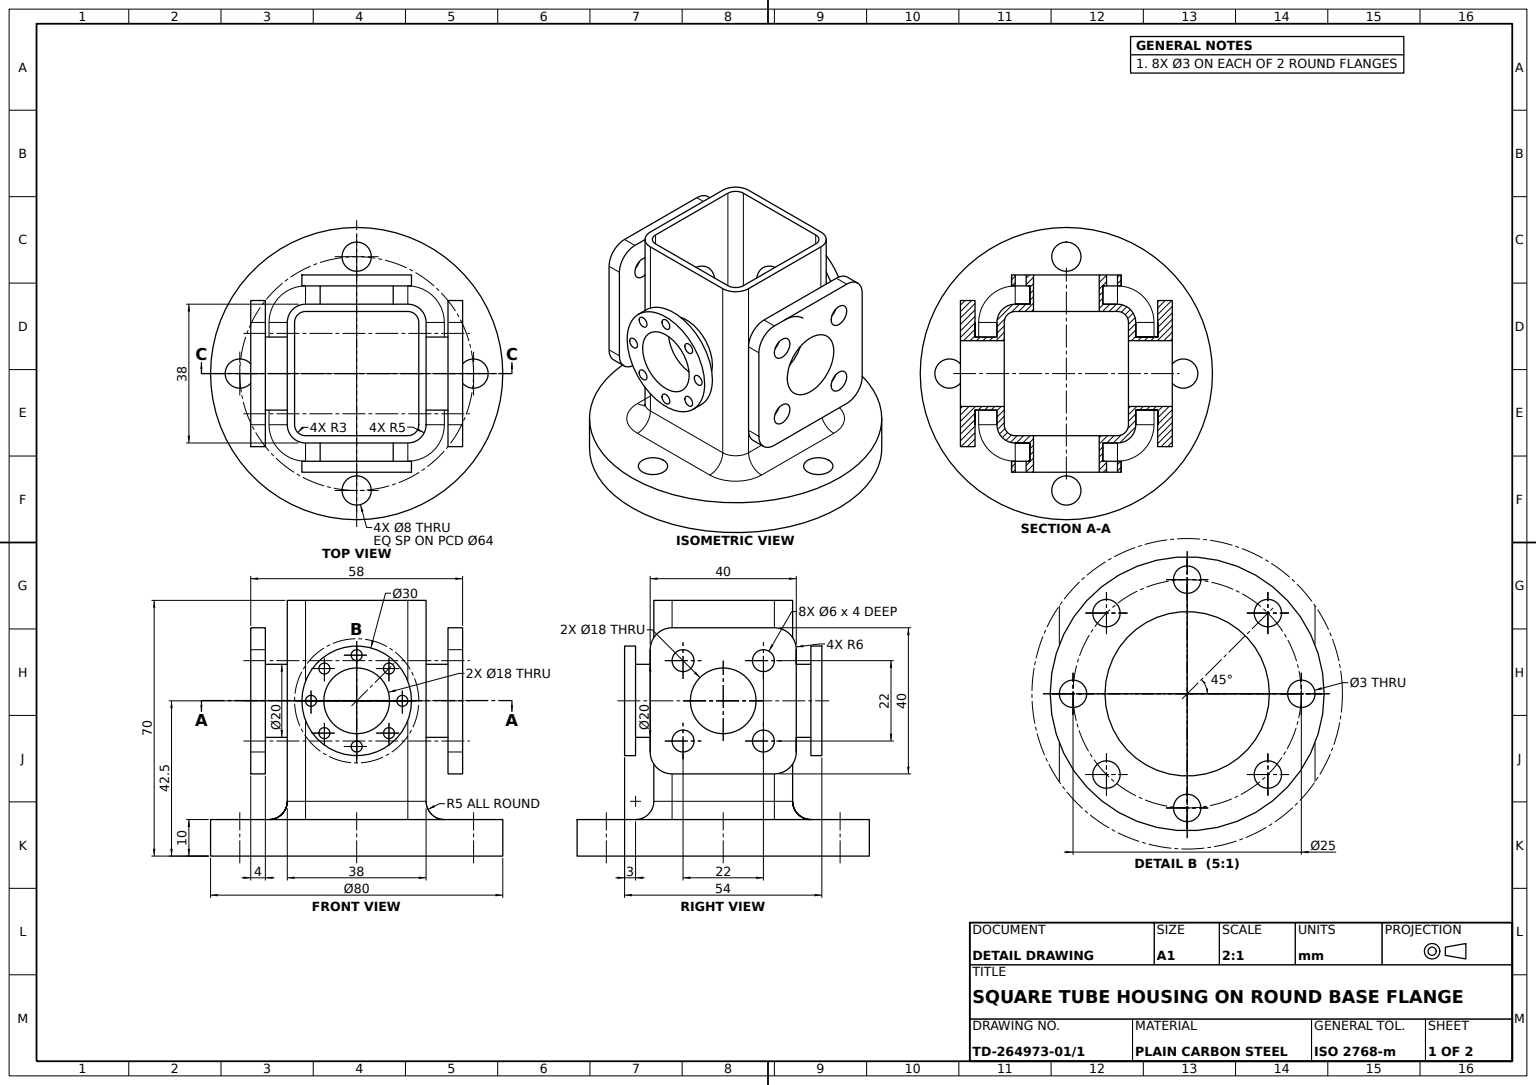
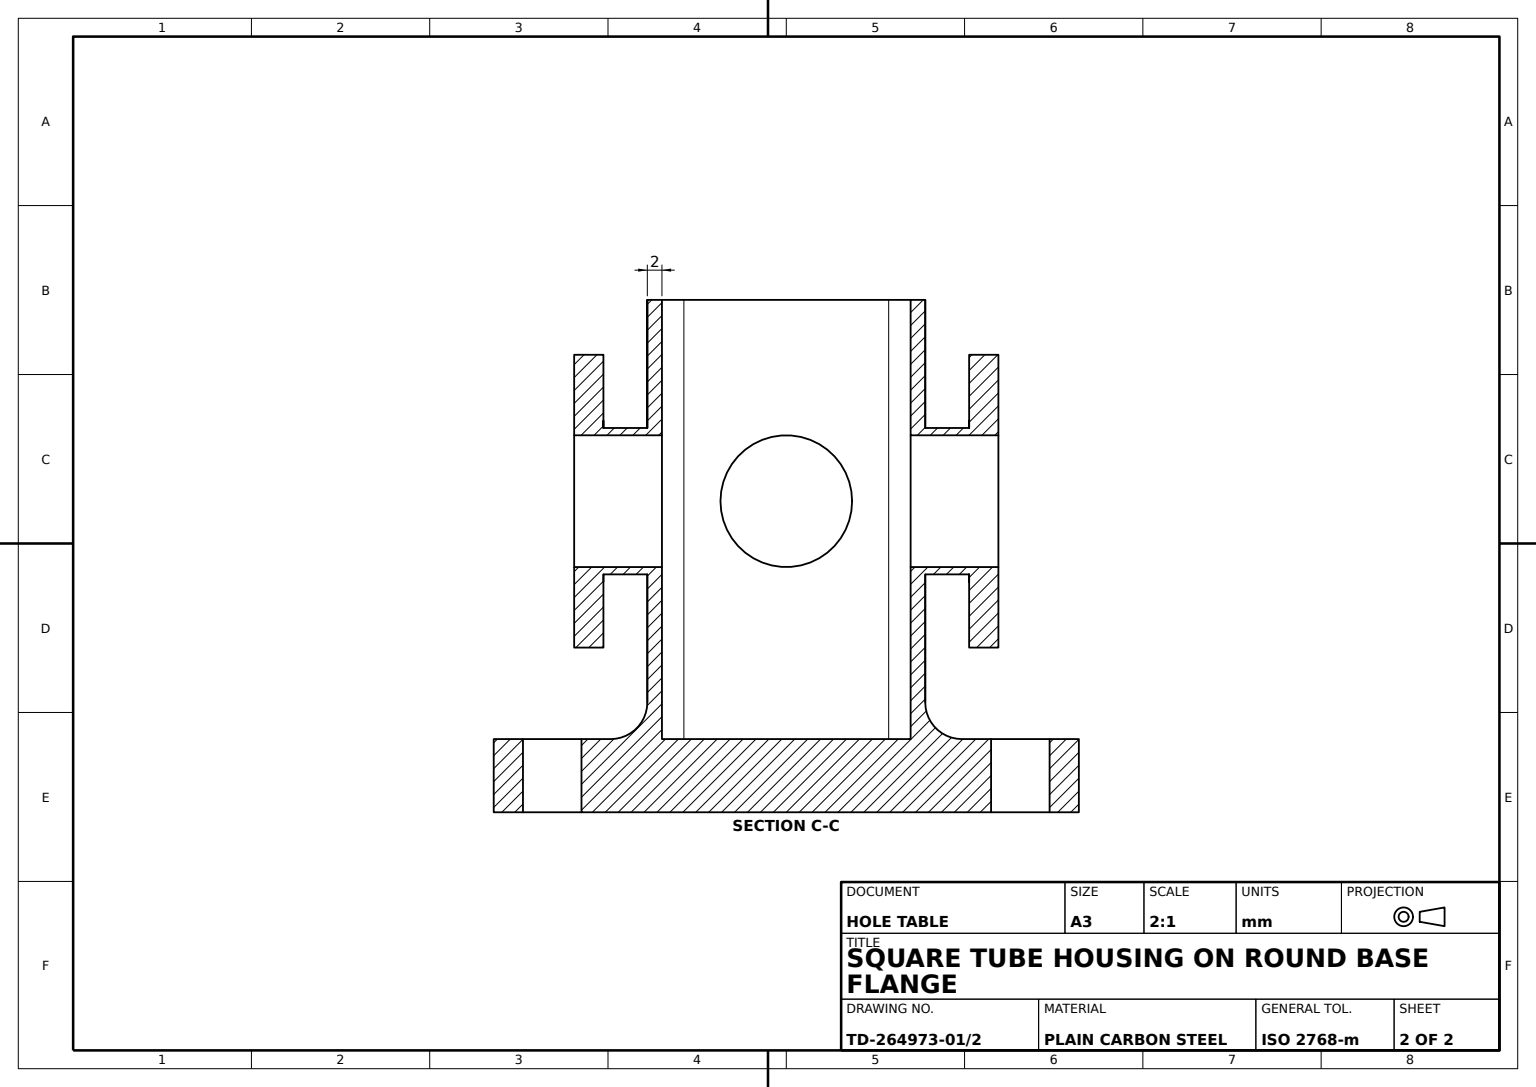
solid
v1 (29,42.5,-9)
v2 (29,42.5,9)
e1 v1 v2 CIRCLE(AX(P(29,42.5,0),D(1,0,0),D(0,0,-1)),9)
v3 (17,42.5,9)
e2 v2 v3 LINE
v4 (17,42.5,-9)
e3 v3 v4 CIRCLE(AX(P(17,42.5,0),D(-1,0,0),D(0,0,1)),9)
e4 v1 v4 LINE
face CYL(AX(P(41,42.5,0),D(-1,0,0),D(0,0,1)),9) rev [e1 e2 e3 -e4]
v5 (1.5,55,-27)
v6 (1.5,55,-24)
e5 v5 v6 LINE
v7 (-1.5,55,-24)
e6 v7 v6 CIRCLE(AX(P(0,55,-24),D(0,0,-1),D(-1,0,0)),1.5)
v8 (-1.5,55,-27)
e7 v8 v7 LINE
e8 v8 v5 CIRCLE(AX(P(0,55,-27),D(0,0,-1),D(-1,0,0)),1.5)
face CYL(AX(P(0,55,-27),D(0,0,1),D(1,0,0)),1.5) rev [e5 -e6 -e7 e8]
v9 (7.338835,51.338835,27)
v10 (7.338835,51.338835,24)
e9 v9 v10 LINE
v11 (10.338835,51.338835,24)
e10 v11 v10 CIRCLE(AX(P(8.838835,51.338835,24),D(0,0,1),D(1,0,0)),1.5)
v12 (10.338835,51.338835,27)
e11 v12 v11 LINE
e12 v12 v9 CIRCLE(AX(P(8.838835,51.338835,27),D(0,0,1),D(1,0,0)),1.5)
face CYL(AX(P(8.838835,51.338835,27),D(0,0,-1),D(-1,0,0)),1.5) rev [e9 -e10 -e11 e12]
v13 (-17,70,-14)
v14 (-17,70,14)
e13 v13 v14 LINE
v15 (-17,10,14)
e14 v14 v15 LINE
v16 (-17,10,-14)
e15 v16 v15 LINE
e16 v13 v16 LINE
v17 (-17,42.5,-9)
v18 (-17,42.5,9)
e17 v17 v18 CIRCLE(AX(P(-17,42.5,0),D(1,0,0),D(0,0,-1)),9)
e18 v18 v17 CIRCLE(AX(P(-17,42.5,0),D(1,0,0),D(0,0,-1)),9)
face PLANE(AX(P(-17,70,-14),D(1,0,0),D(0,0,-1))) [e13 e14 -e15 -e16] [-e17 -e18]
v19 (-25,62.5,-14)
v20 (-25,56.5,-20)
e19 v19 v20 CIRCLE(AX(P(-25,56.5,-14),D(-1,0,0),D(0,0,1)),6)
v21 (-29,56.5,-20)
e20 v21 v20 LINE
v22 (-29,62.5,-14)
e21 v22 v21 CIRCLE(AX(P(-29,56.5,-14),D(-1,0,0),D(0,0,1)),6)
e22 v22 v19 LINE
face CYL(AX(P(-29,56.5,-14),D(1,0,0),D(0,0,-1)),6) [e19 -e20 -e21 e22]
v23 (-1.5,30,-24)
v24 (1.5,30,-24)
e23 v23 v24 CIRCLE(AX(P(0,30,-24),D(0,0,-1),D(-1,0,0)),1.5)
v25 (-1.5,30,-27)
e24 v25 v23 LINE
v26 (1.5,30,-27)
e25 v25 v26 CIRCLE(AX(P(0,30,-27),D(0,0,-1),D(-1,0,0)),1.5)
e26 v26 v24 LINE
face CYL(AX(P(0,30,-27),D(0,0,1),D(1,0,0)),1.5) rev [-e23 -e24 e25 e26]
v27 (-25,42.5,-10)
v28 (-19,42.5,-10)
e27 v27 v28 LINE
v29 (-25,42.5,10)
e28 v29 v27 CIRCLE(AX(P(-25,42.5,0),D(-1,0,0),D(0,0,1)),10)
v30 (-19,42.5,10)
e29 v29 v30 LINE
e30 v30 v28 CIRCLE(AX(P(-19,42.5,0),D(-1,0,0),D(0,0,-1)),10)
face CYL(AX(P(-25,42.5,0),D(1,0,0),D(0,0,-1)),10) [-e27 -e28 e29 e30]
v31 (0,10,40)
v32 (0,0,40)
e31 v31 v32 LINE
v33 (0,0,-40)
e32 v32 v33 CIRCLE(AX(P(0,0,0),D(0,1,0),D(0,0,1)),40)
v34 (0,10,-40)
e33 v34 v33 LINE
e34 v31 v34 CIRCLE(AX(P(0,10,0),D(0,1,0),D(0,0,1)),40)
face CYL(AX(P(0,10,0),D(0,-1,0),D(0,0,-1)),40) [e31 e32 -e33 -e34]
v35 (0,10,28)
v36 (0,10,36)
e35 v35 v36 CIRCLE(AX(P(0,10,32),D(0,1,0),D(0,0,1)),4)
v37 (0,0,36)
e36 v36 v37 LINE
v38 (0,0,28)
e37 v38 v37 CIRCLE(AX(P(0,0,32),D(0,1,0),D(0,0,1)),4)
e38 v35 v38 LINE
face CYL(AX(P(0,10,32),D(0,-1,0),D(0,0,-1)),4) rev [e35 e36 -e37 -e38]
v39 (1.5,30,27)
v40 (1.5,30,24)
e39 v39 v40 LINE
v41 (-1.5,30,27)
e40 v39 v41 CIRCLE(AX(P(0,30,27),D(0,0,1),D(1,0,0)),1.5)
v42 (-1.5,30,24)
e41 v41 v42 LINE
e42 v40 v42 CIRCLE(AX(P(0,30,24),D(0,0,1),D(1,0,0)),1.5)
face CYL(AX(P(0,30,27),D(0,0,-1),D(-1,0,0)),1.5) rev [-e39 e40 e41 -e42]
v43 (-14,10,-17)
e43 v43 v16 CIRCLE(AX(P(-14,10,-14),D(0,1,0),D(1,0,0)),3)
v44 (-14,70,-17)
e44 v44 v43 LINE
e45 v44 v13 CIRCLE(AX(P(-14,70,-14),D(0,1,0),D(1,0,0)),3)
face CYL(AX(P(-14,70,-14),D(0,-1,0),D(0,0,-1)),3) rev [-e43 -e44 e45 e16]
v45 (29,62.5,14)
v46 (29,56.5,20)
e46 v45 v46 CIRCLE(AX(P(29,56.5,14),D(1,0,0),D(0,0,-1)),6)
v47 (25,62.5,14)
e47 v45 v47 LINE
v48 (25,56.5,20)
e48 v47 v48 CIRCLE(AX(P(25,56.5,14),D(1,0,0),D(0,0,-1)),6)
e49 v46 v48 LINE
face CYL(AX(P(29,56.5,14),D(-1,0,0),D(0,0,1)),6) [-e46 e47 e48 -e49]
v49 (-14,42.5,27)
v50 (-11,42.5,27)
e50 v49 v50 CIRCLE(AX(P(-12.5,42.5,27),D(0,0,1),D(1,0,0)),1.5)
v51 (-11,42.5,24)
e51 v50 v51 LINE
v52 (-14,42.5,24)
e52 v52 v51 CIRCLE(AX(P(-12.5,42.5,24),D(0,0,1),D(1,0,0)),1.5)
e53 v49 v52 LINE
face CYL(AX(P(-12.5,42.5,27),D(0,0,-1),D(-1,0,0)),1.5) rev [e50 e51 -e52 -e53]
v53 (-7.338835,51.338835,27)
v54 (-10.338835,51.338835,27)
e54 v53 v54 CIRCLE(AX(P(-8.838835,51.338835,27),D(0,0,1),D(1,0,0)),1.5)
v55 (-10.338835,51.338835,24)
e55 v54 v55 LINE
v56 (-7.338835,51.338835,24)
e56 v56 v55 CIRCLE(AX(P(-8.838835,51.338835,24),D(0,0,1),D(1,0,0)),1.5)
e57 v53 v56 LINE
face CYL(AX(P(-8.838835,51.338835,27),D(0,0,-1),D(-1,0,0)),1.5) rev [e54 e55 -e56 -e57]
v57 (11,42.5,-27)
v58 (11,42.5,-24)
e58 v57 v58 LINE
v59 (14,42.5,-24)
e59 v59 v58 CIRCLE(AX(P(12.5,42.5,-24),D(0,0,-1),D(-1,0,0)),1.5)
v60 (14,42.5,-27)
e60 v60 v59 LINE
e61 v60 v57 CIRCLE(AX(P(12.5,42.5,-27),D(0,0,-1),D(-1,0,0)),1.5)
face CYL(AX(P(12.5,42.5,-27),D(0,0,1),D(1,0,0)),1.5) rev [e58 -e59 -e60 e61]
v61 (-25,28.5,-20)
v62 (-25,22.5,-14)
e62 v61 v62 CIRCLE(AX(P(-25,28.5,-14),D(-1,0,0),D(0,0,1)),6)
v63 (-29,22.5,-14)
e63 v63 v62 LINE
v64 (-29,28.5,-20)
e64 v64 v63 CIRCLE(AX(P(-29,28.5,-14),D(-1,0,0),D(0,0,1)),6)
e65 v64 v61 LINE
face CYL(AX(P(-29,28.5,-14),D(1,0,0),D(0,0,-1)),6) [e62 -e63 -e64 e65]
v65 (29,53.5,14)
v66 (29,53.5,8)
e66 v65 v66 CIRCLE(AX(P(29,53.5,11),D(1,0,0),D(0,0,-1)),3)
v67 (25,53.5,8)
e67 v66 v67 LINE
v68 (25,53.5,14)
e68 v68 v67 CIRCLE(AX(P(25,53.5,11),D(1,0,0),D(0,0,-1)),3)
e69 v65 v68 LINE
face CYL(AX(P(29,53.5,11),D(-1,0,0),D(0,0,1)),3) rev [e66 e67 -e68 -e69]
v69 (25,28.5,20)
e70 v48 v69 LINE
v70 (29,28.5,20)
e71 v70 v69 LINE
e72 v46 v70 LINE
face PLANE(AX(P(29,56.5,20),D(0,0,-1),D(-1,0,0))) rev [e49 e70 -e71 -e72]
v71 (-25,28.5,20)
v72 (-25,56.5,20)
e73 v71 v72 LINE
v73 (-29,56.5,20)
e74 v73 v72 LINE
v74 (-29,28.5,20)
e75 v74 v73 LINE
e76 v74 v71 LINE
face PLANE(AX(P(-29,56.5,20),D(0,0,-1),D(-1,0,0))) rev [e73 -e74 -e75 e76]
v75 (-7.338835,33.661165,27)
v76 (-7.338835,33.661165,24)
e77 v75 v76 LINE
v77 (-10.338835,33.661165,24)
e78 v77 v76 CIRCLE(AX(P(-8.838835,33.661165,24),D(0,0,1),D(1,0,0)),1.5)
v78 (-10.338835,33.661165,27)
e79 v78 v77 LINE
e80 v78 v75 CIRCLE(AX(P(-8.838835,33.661165,27),D(0,0,1),D(1,0,0)),1.5)
face CYL(AX(P(-8.838835,33.661165,27),D(0,0,-1),D(-1,0,0)),1.5) rev [e77 -e78 -e79 e80]
v79 (-29,53.5,14)
v80 (-25,53.5,14)
e81 v79 v80 LINE
v81 (-25,53.5,8)
e82 v81 v80 CIRCLE(AX(P(-25,53.5,11),D(-1,0,0),D(0,0,1)),3)
v82 (-29,53.5,8)
e83 v82 v81 LINE
e84 v82 v79 CIRCLE(AX(P(-29,53.5,11),D(-1,0,0),D(0,0,1)),3)
face CYL(AX(P(-29,53.5,11),D(1,0,0),D(0,0,-1)),3) rev [e81 -e82 -e83 e84]
v83 (7.338835,33.661165,27)
v84 (10.338835,33.661165,27)
e85 v83 v84 CIRCLE(AX(P(8.838835,33.661165,27),D(0,0,1),D(1,0,0)),1.5)
v85 (10.338835,33.661165,24)
e86 v84 v85 LINE
v86 (7.338835,33.661165,24)
e87 v86 v85 CIRCLE(AX(P(8.838835,33.661165,24),D(0,0,1),D(1,0,0)),1.5)
e88 v83 v86 LINE
face CYL(AX(P(8.838835,33.661165,27),D(0,0,-1),D(-1,0,0)),1.5) rev [e85 e86 -e87 -e88]
v87 (19,70,14)
v88 (19,15,14)
e89 v87 v88 LINE
v89 (19,15,-14)
e90 v88 v89 LINE
v90 (19,70,-14)
e91 v90 v89 LINE
e92 v87 v90 LINE
v91 (19,42.5,10)
v92 (19,42.5,-10)
e93 v91 v92 CIRCLE(AX(P(19,42.5,0),D(1,0,0),D(0,0,1)),10)
e94 v92 v91 CIRCLE(AX(P(19,42.5,0),D(1,0,0),D(0,0,1)),10)
face PLANE(AX(P(19,70,-14),D(-1,0,0),D(0,0,1))) rev [e89 e90 -e91 -e92] [-e93 -e94]
v93 (14,10,24)
v94 (-14,10,24)
e95 v93 v94 LINE
v95 (14,15,19)
e96 v93 v95 CIRCLE(AX(P(14,15,24),D(1,0,0),D(0,0,-1)),5)
v96 (-14,15,19)
e97 v96 v95 LINE
e98 v94 v96 CIRCLE(AX(P(-14,15,24),D(1,0,0),D(0,0,-1)),5)
face CYL(AX(P(-14,15,24),D(1,0,0),D(0,0,-1)),5) rev [-e95 e96 -e97 -e98]
e99 v84 v83 CIRCLE(AX(P(8.838835,33.661165,27),D(0,0,1),D(1,0,0)),1.5)
e100 v85 v86 CIRCLE(AX(P(8.838835,33.661165,24),D(0,0,1),D(1,0,0)),1.5)
face CYL(AX(P(8.838835,33.661165,27),D(0,0,-1),D(-1,0,0)),1.5) rev [e99 e88 -e100 -e86]
v97 (-9,42.5,27)
v98 (9,42.5,27)
e101 v97 v98 CIRCLE(AX(P(0,42.5,27),D(0,0,1),D(1,0,0)),9)
v99 (9,42.5,17)
e102 v99 v98 LINE
v100 (-9,42.5,17)
e103 v99 v100 CIRCLE(AX(P(0,42.5,17),D(0,0,-1),D(-1,0,0)),9)
e104 v100 v97 LINE
face CYL(AX(P(0,42.5,-41),D(0,0,1),D(1,0,0)),9) rev [e101 -e102 e103 e104]
v101 (7.338835,51.338835,-27)
v102 (10.338835,51.338835,-27)
e105 v101 v102 CIRCLE(AX(P(8.838835,51.338835,-27),D(0,0,-1),D(-1,0,0)),1.5)
e106 v102 v101 CIRCLE(AX(P(8.838835,51.338835,-27),D(0,0,-1),D(-1,0,0)),1.5)
v103 (15,42.5,-27)
v104 (-15,42.5,-27)
e107 v103 v104 CIRCLE(AX(P(0,42.5,-27),D(0,0,-1),D(-1,0,0)),15)
e108 v104 v103 CIRCLE(AX(P(0,42.5,-27),D(0,0,-1),D(-1,0,0)),15)
e109 v57 v60 CIRCLE(AX(P(12.5,42.5,-27),D(0,0,-1),D(-1,0,0)),1.5)
e110 v26 v25 CIRCLE(AX(P(0,30,-27),D(0,0,-1),D(-1,0,0)),1.5)
v105 (-11,42.5,-27)
v106 (-14,42.5,-27)
e111 v105 v106 CIRCLE(AX(P(-12.5,42.5,-27),D(0,0,-1),D(-1,0,0)),1.5)
e112 v106 v105 CIRCLE(AX(P(-12.5,42.5,-27),D(0,0,-1),D(-1,0,0)),1.5)
v107 (-10.338835,51.338835,-27)
v108 (-7.338835,51.338835,-27)
e113 v107 v108 CIRCLE(AX(P(-8.838835,51.338835,-27),D(0,0,-1),D(-1,0,0)),1.5)
e114 v108 v107 CIRCLE(AX(P(-8.838835,51.338835,-27),D(0,0,-1),D(-1,0,0)),1.5)
e115 v5 v8 CIRCLE(AX(P(0,55,-27),D(0,0,-1),D(-1,0,0)),1.5)
v109 (-9,42.5,-27)
v110 (9,42.5,-27)
e116 v109 v110 CIRCLE(AX(P(0,42.5,-27),D(0,0,-1),D(-1,0,0)),9)
e117 v110 v109 CIRCLE(AX(P(0,42.5,-27),D(0,0,-1),D(-1,0,0)),9)
v111 (-10.338835,33.661165,-27)
v112 (-7.338835,33.661165,-27)
e118 v111 v112 CIRCLE(AX(P(-8.838835,33.661165,-27),D(0,0,-1),D(-1,0,0)),1.5)
e119 v112 v111 CIRCLE(AX(P(-8.838835,33.661165,-27),D(0,0,-1),D(-1,0,0)),1.5)
v113 (7.338835,33.661165,-27)
v114 (10.338835,33.661165,-27)
e120 v113 v114 CIRCLE(AX(P(8.838835,33.661165,-27),D(0,0,-1),D(-1,0,0)),1.5)
e121 v114 v113 CIRCLE(AX(P(8.838835,33.661165,-27),D(0,0,-1),D(-1,0,0)),1.5)
face PLANE(AX(P(0,42.5,-27),D(0,0,-1),D(-1,0,0))) [-e105 -e106] [e107 e108] [-e109 -e61] [-e110 -e25] [-e111 -e112] [-e113 -e114] [-e8 -e115] [-e116 -e117] [-e118 -e119] [-e120 -e121]
v115 (15,42.5,-24)
e122 v103 v115 LINE
v116 (-15,42.5,-24)
e123 v115 v116 CIRCLE(AX(P(0,42.5,-24),D(0,0,-1),D(-1,0,0)),15)
e124 v104 v116 LINE
face CYL(AX(P(0,42.5,-27),D(0,0,1),D(1,0,0)),15) [-e107 e122 e123 -e124]
e125 v116 v115 CIRCLE(AX(P(0,42.5,-24),D(0,0,-1),D(-1,0,0)),15)
face CYL(AX(P(0,42.5,-27),D(0,0,1),D(1,0,0)),15) [-e108 e124 e125 -e122]
v117 (7.338835,51.338835,-24)
e126 v101 v117 LINE
v118 (10.338835,51.338835,-24)
e127 v118 v117 CIRCLE(AX(P(8.838835,51.338835,-24),D(0,0,-1),D(-1,0,0)),1.5)
e128 v102 v118 LINE
face CYL(AX(P(8.838835,51.338835,-27),D(0,0,1),D(1,0,0)),1.5) rev [e126 -e127 -e128 e106]
v119 (10.338835,33.661165,-24)
v120 (7.338835,33.661165,-24)
e129 v119 v120 CIRCLE(AX(P(8.838835,33.661165,-24),D(0,0,-1),D(-1,0,0)),1.5)
e130 v114 v119 LINE
e131 v113 v120 LINE
face CYL(AX(P(8.838835,33.661165,-27),D(0,0,1),D(1,0,0)),1.5) rev [-e129 -e130 e121 e131]
e132 v6 v7 CIRCLE(AX(P(0,55,-24),D(0,0,-1),D(-1,0,0)),1.5)
face CYL(AX(P(0,55,-27),D(0,0,1),D(1,0,0)),1.5) rev [e115 e7 -e132 -e5]
e133 v4 v3 CIRCLE(AX(P(17,42.5,0),D(-1,0,0),D(0,0,1)),9)
e134 v2 v1 CIRCLE(AX(P(29,42.5,0),D(1,0,0),D(0,0,-1)),9)
face CYL(AX(P(41,42.5,0),D(-1,0,0),D(0,0,1)),9) rev [e4 e133 -e2 e134]
v121 (29,31.5,14)
v122 (25,31.5,14)
e135 v121 v122 LINE
v123 (25,31.5,8)
e136 v123 v122 CIRCLE(AX(P(25,31.5,11),D(1,0,0),D(0,0,-1)),3)
v124 (29,31.5,8)
e137 v124 v123 LINE
e138 v124 v121 CIRCLE(AX(P(29,31.5,11),D(1,0,0),D(0,0,-1)),3)
face CYL(AX(P(29,31.5,11),D(-1,0,0),D(0,0,1)),3) rev [e135 -e136 -e137 e138]
v125 (-10.338835,33.661165,-24)
e139 v111 v125 LINE
v126 (-7.338835,33.661165,-24)
e140 v112 v126 LINE
e141 v125 v126 CIRCLE(AX(P(-8.838835,33.661165,-24),D(0,0,-1),D(-1,0,0)),1.5)
face CYL(AX(P(-8.838835,33.661165,-27),D(0,0,1),D(1,0,0)),1.5) rev [-e139 e118 e140 -e141]
e142 v67 v68 CIRCLE(AX(P(25,53.5,11),D(1,0,0),D(0,0,-1)),3)
e143 v66 v65 CIRCLE(AX(P(29,53.5,11),D(1,0,0),D(0,0,-1)),3)
face CYL(AX(P(29,53.5,11),D(-1,0,0),D(0,0,1)),3) rev [e69 -e142 -e67 e143]
v127 (-29,53.5,-14)
v128 (-29,53.5,-8)
e144 v127 v128 CIRCLE(AX(P(-29,53.5,-11),D(-1,0,0),D(0,0,1)),3)
e145 v128 v127 CIRCLE(AX(P(-29,53.5,-11),D(-1,0,0),D(0,0,1)),3)
e146 v79 v82 CIRCLE(AX(P(-29,53.5,11),D(-1,0,0),D(0,0,1)),3)
v129 (-29,31.5,-8)
v130 (-29,31.5,-14)
e147 v129 v130 CIRCLE(AX(P(-29,31.5,-11),D(-1,0,0),D(0,0,1)),3)
e148 v130 v129 CIRCLE(AX(P(-29,31.5,-11),D(-1,0,0),D(0,0,1)),3)
v131 (-29,62.5,14)
e149 v131 v22 LINE
e150 v21 v64 LINE
v132 (-29,22.5,14)
e151 v63 v132 LINE
e152 v132 v74 CIRCLE(AX(P(-29,28.5,14),D(-1,0,0),D(0,0,1)),6)
e153 v73 v131 CIRCLE(AX(P(-29,56.5,14),D(-1,0,0),D(0,0,-1)),6)
v133 (-29,31.5,14)
v134 (-29,31.5,8)
e154 v133 v134 CIRCLE(AX(P(-29,31.5,11),D(-1,0,0),D(0,0,1)),3)
e155 v134 v133 CIRCLE(AX(P(-29,31.5,11),D(-1,0,0),D(0,0,1)),3)
v135 (-29,42.5,9)
v136 (-29,42.5,-9)
e156 v135 v136 CIRCLE(AX(P(-29,42.5,0),D(-1,0,0),D(0,0,1)),9)
e157 v136 v135 CIRCLE(AX(P(-29,42.5,0),D(-1,0,0),D(0,0,1)),9)
face PLANE(AX(P(-29,28.5,-14),D(-1,0,0),D(0,0,1))) [-e144 -e145] [-e146 -e84] [-e147 -e148] [e149 e21 e150 e64 e151 e152 e75 e153] [-e154 -e155] [-e156 -e157]
e158 v98 v97 CIRCLE(AX(P(0,42.5,27),D(0,0,1),D(1,0,0)),9)
e159 v41 v39 CIRCLE(AX(P(0,30,27),D(0,0,1),D(1,0,0)),1.5)
e160 v50 v49 CIRCLE(AX(P(-12.5,42.5,27),D(0,0,1),D(1,0,0)),1.5)
v137 (1.5,55,27)
v138 (-1.5,55,27)
e161 v137 v138 CIRCLE(AX(P(0,55,27),D(0,0,1),D(1,0,0)),1.5)
e162 v138 v137 CIRCLE(AX(P(0,55,27),D(0,0,1),D(1,0,0)),1.5)
e163 v9 v12 CIRCLE(AX(P(8.838835,51.338835,27),D(0,0,1),D(1,0,0)),1.5)
e164 v75 v78 CIRCLE(AX(P(-8.838835,33.661165,27),D(0,0,1),D(1,0,0)),1.5)
v139 (-15,42.5,27)
v140 (15,42.5,27)
e165 v139 v140 CIRCLE(AX(P(0,42.5,27),D(0,0,1),D(1,0,0)),15)
e166 v140 v139 CIRCLE(AX(P(0,42.5,27),D(0,0,1),D(1,0,0)),15)
e167 v54 v53 CIRCLE(AX(P(-8.838835,51.338835,27),D(0,0,1),D(1,0,0)),1.5)
v141 (11,42.5,27)
v142 (14,42.5,27)
e168 v141 v142 CIRCLE(AX(P(12.5,42.5,27),D(0,0,1),D(1,0,0)),1.5)
e169 v142 v141 CIRCLE(AX(P(12.5,42.5,27),D(0,0,1),D(1,0,0)),1.5)
face PLANE(AX(P(0,42.5,27),D(0,0,1),D(1,0,0))) [-e158 -e101] [-e159 -e40] [-e160 -e50] [-e161 -e162] [-e163 -e12] [-e164 -e80] [e165 e166] [-e54 -e167] [-e85 -e99] [-e168 -e169]
v143 (-14,10,17)
e170 v15 v143 CIRCLE(AX(P(-14,10,14),D(0,1,0),D(1,0,0)),3)
v144 (-14,70,17)
e171 v14 v144 CIRCLE(AX(P(-14,70,14),D(0,1,0),D(1,0,0)),3)
e172 v144 v143 LINE
face CYL(AX(P(-14,70,14),D(0,-1,0),D(0,0,-1)),3) rev [-e170 -e14 e171 e172]
v145 (-15,42.5,24)
e173 v139 v145 LINE
v146 (15,42.5,24)
e174 v145 v146 CIRCLE(AX(P(0,42.5,24),D(0,0,1),D(1,0,0)),15)
e175 v140 v146 LINE
face CYL(AX(P(0,42.5,27),D(0,0,-1),D(-1,0,0)),15) [e173 e174 -e175 -e165]
v147 (14,70,17)
e176 v144 v147 LINE
v148 (14,10,17)
e177 v147 v148 LINE
e178 v143 v148 LINE
e179 v100 v99 CIRCLE(AX(P(0,42.5,17),D(0,0,-1),D(-1,0,0)),9)
face PLANE(AX(P(-14,70,17),D(0,0,-1),D(-1,0,0))) [-e172 e176 e177 -e178] [-e179 -e103]
e180 v17 v136 LINE
e181 v18 v135 LINE
face CYL(AX(P(41,42.5,0),D(-1,0,0),D(0,0,1)),9) rev [e18 e180 e157 -e181]
v149 (-24,10,14)
e182 v94 v149 CIRCLE(AX(P(-14,10,14),D(0,-1,0),D(0,0,1)),10)
v150 (-19,15,14)
e183 v150 v96 CIRCLE(AX(P(-14,15,14),D(0,1,0),D(0,0,1)),5)
e184 v150 v149 CIRCLE(AX(P(-24,15,14),D(0,0,-1),D(0,1,0)),5)
face TORUS(AX(P(-14,15,14),D(0,1,0),D(0,0,1)),10,5) rev [-e182 e98 -e183 e184]
e185 v10 v11 CIRCLE(AX(P(8.838835,51.338835,24),D(0,0,1),D(1,0,0)),1.5)
e186 v51 v52 CIRCLE(AX(P(-12.5,42.5,24),D(0,0,1),D(1,0,0)),1.5)
e187 v42 v40 CIRCLE(AX(P(0,30,24),D(0,0,1),D(1,0,0)),1.5)
v151 (11,42.5,24)
v152 (14,42.5,24)
e188 v151 v152 CIRCLE(AX(P(12.5,42.5,24),D(0,0,1),D(1,0,0)),1.5)
e189 v152 v151 CIRCLE(AX(P(12.5,42.5,24),D(0,0,1),D(1,0,0)),1.5)
v153 (-10,42.5,24)
v154 (10,42.5,24)
e190 v153 v154 CIRCLE(AX(P(0,42.5,24),D(0,0,1),D(1,0,0)),10)
e191 v154 v153 CIRCLE(AX(P(0,42.5,24),D(0,0,1),D(1,0,0)),10)
v155 (1.5,55,24)
v156 (-1.5,55,24)
e192 v155 v156 CIRCLE(AX(P(0,55,24),D(0,0,1),D(1,0,0)),1.5)
e193 v156 v155 CIRCLE(AX(P(0,55,24),D(0,0,1),D(1,0,0)),1.5)
e194 v76 v77 CIRCLE(AX(P(-8.838835,33.661165,24),D(0,0,1),D(1,0,0)),1.5)
e195 v55 v56 CIRCLE(AX(P(-8.838835,51.338835,24),D(0,0,1),D(1,0,0)),1.5)
e196 v146 v145 CIRCLE(AX(P(0,42.5,24),D(0,0,1),D(1,0,0)),15)
face PLANE(AX(P(0,42.5,24),D(0,0,1),D(1,0,0))) rev [e10 e185] [e186 e52] [e87 e100] [e42 e187] [e188 e189] [e190 e191] [e192 e193] [e78 e194] [e195 e56] [-e174 -e196]
e197 v33 v32 CIRCLE(AX(P(0,0,0),D(0,1,0),D(0,0,1)),40)
e198 v34 v31 CIRCLE(AX(P(0,10,0),D(0,1,0),D(0,0,1)),40)
face CYL(AX(P(0,10,0),D(0,-1,0),D(0,0,-1)),40) [e33 e197 -e31 -e198]
v157 (29,28.5,-20)
v158 (25,28.5,-20)
e199 v157 v158 LINE
v159 (29,22.5,-14)
e200 v159 v157 CIRCLE(AX(P(29,28.5,-14),D(1,0,0),D(0,0,-1)),6)
v160 (25,22.5,-14)
e201 v159 v160 LINE
e202 v160 v158 CIRCLE(AX(P(25,28.5,-14),D(1,0,0),D(0,0,-1)),6)
face CYL(AX(P(29,28.5,-14),D(-1,0,0),D(0,0,1)),6) [-e199 -e200 e201 e202]
e203 v37 v38 CIRCLE(AX(P(0,0,32),D(0,1,0),D(0,0,1)),4)
e204 v36 v35 CIRCLE(AX(P(0,10,32),D(0,1,0),D(0,0,1)),4)
face CYL(AX(P(0,10,32),D(0,-1,0),D(0,0,-1)),4) rev [e38 -e203 -e36 e204]
e205 v95 v88 CIRCLE(AX(P(14,15,14),D(0,1,0),D(0,0,1)),5)
v161 (14,70,19)
e206 v161 v87 CIRCLE(AX(P(14,70,14),D(0,1,0),D(0,0,1)),5)
e207 v161 v95 LINE
face CYL(AX(P(14,70,14),D(0,-1,0),D(0,0,-1)),5) [e205 -e89 -e206 e207]
v162 (-10.338835,51.338835,-24)
v163 (-7.338835,51.338835,-24)
e208 v162 v163 CIRCLE(AX(P(-8.838835,51.338835,-24),D(0,0,-1),D(-1,0,0)),1.5)
e209 v107 v162 LINE
e210 v108 v163 LINE
face CYL(AX(P(-8.838835,51.338835,-27),D(0,0,1),D(1,0,0)),1.5) rev [-e208 -e209 e113 e210]
v164 (29,22.5,14)
v165 (25,22.5,14)
e211 v164 v165 LINE
e212 v165 v160 LINE
e213 v164 v159 LINE
face PLANE(AX(P(29,22.5,14),D(0,1,0),D(0,0,1))) rev [e211 e212 -e201 -e213]
v166 (10,42.5,19)
e214 v154 v166 LINE
v167 (-10,42.5,19)
e215 v166 v167 CIRCLE(AX(P(0,42.5,19),D(0,0,1),D(-1,0,0)),10)
e216 v153 v167 LINE
face CYL(AX(P(0,42.5,24),D(0,0,-1),D(-1,0,0)),10) [e214 e215 -e216 -e191]
v168 (-25,22.5,14)
e217 v62 v168 LINE
e218 v132 v168 LINE
face PLANE(AX(P(-29,22.5,-14),D(0,1,0),D(0,0,1))) rev [e63 e217 -e218 -e151]
v169 (-14,42.5,-24)
e219 v106 v169 LINE
v170 (-11,42.5,-24)
e220 v105 v170 LINE
e221 v169 v170 CIRCLE(AX(P(-12.5,42.5,-24),D(0,0,-1),D(-1,0,0)),1.5)
face CYL(AX(P(-12.5,42.5,-27),D(0,0,1),D(1,0,0)),1.5) rev [-e219 e112 e220 -e221]
v171 (-25,31.5,-14)
e222 v130 v171 LINE
v172 (-25,31.5,-8)
e223 v129 v172 LINE
e224 v171 v172 CIRCLE(AX(P(-25,31.5,-11),D(-1,0,0),D(0,0,1)),3)
face CYL(AX(P(-29,31.5,-11),D(1,0,0),D(0,0,-1)),3) rev [-e222 e148 e223 -e224]
face CYL(AX(P(0,42.5,-41),D(0,0,1),D(1,0,0)),9) rev [-e104 e179 e102 e158]
e225 v70 v164 CIRCLE(AX(P(29,28.5,14),D(1,0,0),D(0,0,-1)),6)
e226 v69 v165 CIRCLE(AX(P(25,28.5,14),D(1,0,0),D(0,0,-1)),6)
face CYL(AX(P(29,28.5,14),D(-1,0,0),D(0,0,1)),6) [-e225 e71 e226 -e211]
v173 (24,10,-14)
e227 v173 v89 CIRCLE(AX(P(24,15,-14),D(0,0,-1),D(-1,0,0)),5)
v174 (14,10,-24)
e228 v174 v173 CIRCLE(AX(P(14,10,-14),D(0,-1,0),D(0,0,1)),10)
v175 (14,15,-19)
e229 v175 v174 CIRCLE(AX(P(14,15,-24),D(1,0,0),D(0,0,-1)),5)
e230 v89 v175 CIRCLE(AX(P(14,15,-14),D(0,1,0),D(0,0,1)),5)
face TORUS(AX(P(14,15,-14),D(0,1,0),D(0,0,1)),10,5) rev [-e227 -e228 -e229 -e230]
v176 (-25,62.5,14)
e231 v72 v176 CIRCLE(AX(P(-25,56.5,14),D(-1,0,0),D(0,0,-1)),6)
e232 v131 v176 LINE
face CYL(AX(P(-29,56.5,14),D(1,0,0),D(0,0,-1)),6) [e74 e231 -e232 -e153]
v177 (-9,42.5,-17)
e233 v109 v177 LINE
v178 (9,42.5,-17)
e234 v177 v178 CIRCLE(AX(P(0,42.5,-17),D(0,0,1),D(1,0,0)),9)
e235 v110 v178 LINE
face CYL(AX(P(0,42.5,-41),D(0,0,1),D(1,0,0)),9) rev [e117 e233 e234 -e235]
face CYL(AX(P(-8.838835,51.338835,27),D(0,0,-1),D(-1,0,0)),1.5) rev [-e55 e167 e57 -e195]
e236 v20 v61 LINE
face PLANE(AX(P(-29,56.5,-20),D(0,0,1),D(1,0,0))) rev [-e65 -e150 e20 e236]
e237 v28 v30 CIRCLE(AX(P(-19,42.5,0),D(-1,0,0),D(0,0,-1)),10)
v179 (-19,70,-14)
v180 (-19,15,-14)
e238 v179 v180 LINE
e239 v180 v150 LINE
v181 (-19,70,14)
e240 v181 v150 LINE
e241 v179 v181 LINE
face PLANE(AX(P(-19,70,-14),D(1,0,0),D(0,0,-1))) rev [-e30 -e237] [e238 e239 -e240 -e241]
v182 (-32,0,-4)
v183 (-32,0,4)
e242 v182 v183 CIRCLE(AX(P(-32,0,0),D(0,1,0),D(0,0,1)),4)
v184 (-32,10,-4)
e243 v184 v182 LINE
v185 (-32,10,4)
e244 v184 v185 CIRCLE(AX(P(-32,10,0),D(0,1,0),D(0,0,1)),4)
e245 v185 v183 LINE
face CYL(AX(P(-32,10,0),D(0,-1,0),D(0,0,-1)),4) rev [-e242 -e243 e244 e245]
v186 (-25,53.5,-14)
e246 v127 v186 LINE
v187 (-25,53.5,-8)
e247 v187 v186 CIRCLE(AX(P(-25,53.5,-11),D(-1,0,0),D(0,0,1)),3)
e248 v128 v187 LINE
face CYL(AX(P(-29,53.5,-11),D(1,0,0),D(0,0,-1)),3) rev [e246 -e247 -e248 e145]
e249 v178 v177 CIRCLE(AX(P(0,42.5,-17),D(0,0,1),D(1,0,0)),9)
face CYL(AX(P(0,42.5,-41),D(0,0,1),D(1,0,0)),9) rev [e249 -e233 e116 e235]
e250 v121 v124 CIRCLE(AX(P(29,31.5,11),D(1,0,0),D(0,0,-1)),3)
v188 (29,53.5,-8)
v189 (29,53.5,-14)
e251 v188 v189 CIRCLE(AX(P(29,53.5,-11),D(1,0,0),D(0,0,-1)),3)
e252 v189 v188 CIRCLE(AX(P(29,53.5,-11),D(1,0,0),D(0,0,-1)),3)
v190 (29,31.5,-14)
v191 (29,31.5,-8)
e253 v190 v191 CIRCLE(AX(P(29,31.5,-11),D(1,0,0),D(0,0,-1)),3)
e254 v191 v190 CIRCLE(AX(P(29,31.5,-11),D(1,0,0),D(0,0,-1)),3)
v192 (29,56.5,-20)
e255 v157 v192 LINE
v193 (29,62.5,-14)
e256 v192 v193 CIRCLE(AX(P(29,56.5,-14),D(1,0,0),D(0,0,1)),6)
e257 v193 v45 LINE
face PLANE(AX(P(29,28.5,14),D(1,0,0),D(0,0,-1))) [-e134 -e1] [-e138 -e250] [-e251 -e252] [-e253 -e254] [e200 e255 e256 e257 e46 e72 e225 e213] [-e66 -e143]
v194 (32,0,-4)
v195 (32,0,4)
e258 v194 v195 CIRCLE(AX(P(32,0,0),D(0,1,0),D(0,0,1)),4)
e259 v195 v194 CIRCLE(AX(P(32,0,0),D(0,1,0),D(0,0,1)),4)
v196 (0,0,-36)
v197 (0,0,-28)
e260 v196 v197 CIRCLE(AX(P(0,0,-32),D(0,1,0),D(0,0,1)),4)
e261 v197 v196 CIRCLE(AX(P(0,0,-32),D(0,1,0),D(0,0,1)),4)
e262 v183 v182 CIRCLE(AX(P(-32,0,0),D(0,1,0),D(0,0,1)),4)
face PLANE(AX(P(0,0,0),D(0,1,0),D(0,0,1))) rev [e37 e203] [e258 e259] [e260 e261] [e262 e242] [-e32 -e197]
v198 (25,56.5,-20)
e263 v192 v198 LINE
v199 (25,62.5,-14)
e264 v198 v199 CIRCLE(AX(P(25,56.5,-14),D(1,0,0),D(0,0,1)),6)
e265 v193 v199 LINE
face CYL(AX(P(29,56.5,-14),D(-1,0,0),D(0,0,1)),6) [-e256 e263 e264 -e265]
v200 (-24,10,-14)
v201 (-14,10,-24)
e266 v200 v201 CIRCLE(AX(P(-14,10,-14),D(0,-1,0),D(0,0,1)),10)
e267 v180 v200 CIRCLE(AX(P(-24,15,-14),D(0,0,-1),D(-1,0,0)),5)
v202 (-14,15,-19)
e268 v202 v180 CIRCLE(AX(P(-14,15,-14),D(0,1,0),D(0,0,1)),5)
e269 v202 v201 CIRCLE(AX(P(-14,15,-24),D(1,0,0),D(0,0,-1)),5)
face TORUS(AX(P(-14,15,-14),D(0,1,0),D(0,0,1)),10,5) rev [-e266 -e267 -e268 e269]
v203 (25,42.5,-10)
v204 (25,42.5,10)
e270 v203 v204 CIRCLE(AX(P(25,42.5,0),D(1,0,0),D(0,0,-1)),10)
e271 v203 v92 LINE
e272 v204 v91 LINE
face CYL(AX(P(25,42.5,0),D(-1,0,0),D(0,0,1)),10) [-e270 e271 e94 -e272]
v205 (-14,70,-19)
e273 v205 v179 CIRCLE(AX(P(-14,70,-14),D(0,1,0),D(0,0,1)),5)
v206 (-14,70,19)
e274 v181 v206 CIRCLE(AX(P(-14,70,14),D(0,1,0),D(0,0,1)),5)
e275 v206 v161 LINE
v207 (14,70,-19)
e276 v90 v207 CIRCLE(AX(P(14,70,-14),D(0,1,0),D(0,0,-1)),5)
e277 v207 v205 LINE
v208 (17,70,14)
e278 v147 v208 CIRCLE(AX(P(14,70,14),D(0,1,0),D(1,0,0)),3)
v209 (14,70,-17)
e279 v209 v44 LINE
v210 (17,70,-14)
e280 v210 v209 CIRCLE(AX(P(14,70,-14),D(0,1,0),D(1,0,0)),3)
e281 v208 v210 LINE
face PLANE(AX(P(14,70,14),D(0,1,0),D(0,0,1))) [e273 e241 e274 e275 e206 e92 e276 e277] [-e278 -e176 -e171 -e13 -e45 -e279 -e280 -e281]
e282 v137 v155 LINE
e283 v138 v156 LINE
face CYL(AX(P(0,55,27),D(0,0,-1),D(-1,0,0)),1.5) rev [-e282 e161 e283 -e192]
e284 v163 v162 CIRCLE(AX(P(-8.838835,51.338835,-24),D(0,0,-1),D(-1,0,0)),1.5)
v211 (10,42.5,-24)
v212 (-10,42.5,-24)
e285 v211 v212 CIRCLE(AX(P(0,42.5,-24),D(0,0,-1),D(-1,0,0)),10)
e286 v212 v211 CIRCLE(AX(P(0,42.5,-24),D(0,0,-1),D(-1,0,0)),10)
e287 v24 v23 CIRCLE(AX(P(0,30,-24),D(0,0,-1),D(-1,0,0)),1.5)
e288 v117 v118 CIRCLE(AX(P(8.838835,51.338835,-24),D(0,0,-1),D(-1,0,0)),1.5)
e289 v120 v119 CIRCLE(AX(P(8.838835,33.661165,-24),D(0,0,-1),D(-1,0,0)),1.5)
e290 v170 v169 CIRCLE(AX(P(-12.5,42.5,-24),D(0,0,-1),D(-1,0,0)),1.5)
e291 v126 v125 CIRCLE(AX(P(-8.838835,33.661165,-24),D(0,0,-1),D(-1,0,0)),1.5)
e292 v58 v59 CIRCLE(AX(P(12.5,42.5,-24),D(0,0,-1),D(-1,0,0)),1.5)
face PLANE(AX(P(0,42.5,-24),D(0,0,-1),D(-1,0,0))) rev [e208 e284] [e285 e286] [e23 e287] [e288 e127] [e129 e289] [e221 e290] [-e123 -e125] [e132 e6] [e291 e141] [e59 e292]
face CYL(AX(P(0,30,-27),D(0,0,1),D(1,0,0)),1.5) rev [-e287 -e26 e110 e24]
v213 (25,53.5,-8)
e293 v188 v213 LINE
v214 (25,53.5,-14)
e294 v189 v214 LINE
e295 v213 v214 CIRCLE(AX(P(25,53.5,-11),D(1,0,0),D(0,0,-1)),3)
face CYL(AX(P(29,53.5,-11),D(-1,0,0),D(0,0,1)),3) rev [-e293 e251 e294 -e295]
e296 v199 v47 LINE
face PLANE(AX(P(29,62.5,14),D(0,-1,0),D(0,0,-1))) rev [e296 -e47 -e257 e265]
face CYL(AX(P(0,42.5,27),D(0,0,-1),D(-1,0,0)),15) [-e166 e175 e196 -e173]
v215 (0,10,-28)
v216 (0,10,-36)
e297 v215 v216 CIRCLE(AX(P(0,10,-32),D(0,1,0),D(0,0,1)),4)
e298 v216 v196 LINE
e299 v215 v197 LINE
face CYL(AX(P(0,10,-32),D(0,-1,0),D(0,0,-1)),4) rev [e297 e298 -e261 -e299]
face CYL(AX(P(8.838835,51.338835,27),D(0,0,-1),D(-1,0,0)),1.5) rev [e11 -e185 -e9 e163]
v217 (-25,31.5,8)
v218 (-25,31.5,14)
e300 v217 v218 CIRCLE(AX(P(-25,31.5,11),D(-1,0,0),D(0,0,1)),3)
e301 v134 v217 LINE
e302 v133 v218 LINE
face CYL(AX(P(-29,31.5,11),D(1,0,0),D(0,0,-1)),3) rev [-e300 -e301 e155 e302]
v219 (14,10,-17)
e303 v209 v219 LINE
v220 (17,10,-14)
e304 v220 v219 CIRCLE(AX(P(14,10,-14),D(0,1,0),D(1,0,0)),3)
e305 v210 v220 LINE
face CYL(AX(P(14,70,-14),D(0,-1,0),D(0,0,-1)),3) rev [e303 -e304 -e305 e280]
face CYL(AX(P(-8.838835,51.338835,-27),D(0,0,1),D(1,0,0)),1.5) rev [e209 -e284 -e210 e114]
e306 v207 v175 LINE
face CYL(AX(P(14,70,-14),D(0,-1,0),D(0,0,-1)),5) [e230 -e306 -e276 e91]
v221 (17,10,14)
e307 v208 v221 LINE
e308 v148 v221 CIRCLE(AX(P(14,10,14),D(0,1,0),D(1,0,0)),3)
face CYL(AX(P(14,70,14),D(0,-1,0),D(0,0,-1)),3) rev [e278 e307 -e308 -e177]
e309 v186 v187 CIRCLE(AX(P(-25,53.5,-11),D(-1,0,0),D(0,0,1)),3)
face CYL(AX(P(-29,53.5,-11),D(1,0,0),D(0,0,-1)),3) rev [-e246 e144 e248 -e309]
v222 (24,10,14)
e310 v222 v93 CIRCLE(AX(P(14,10,14),D(0,-1,0),D(0,0,1)),10)
e311 v222 v88 CIRCLE(AX(P(24,15,14),D(0,0,-1),D(-1,0,0)),5)
face TORUS(AX(P(14,15,14),D(0,1,0),D(0,0,1)),10,5) rev [-e310 e311 -e205 -e96]
e312 v122 v123 CIRCLE(AX(P(25,31.5,11),D(1,0,0),D(0,0,-1)),3)
face CYL(AX(P(29,31.5,11),D(-1,0,0),D(0,0,1)),3) rev [e137 -e312 -e135 e250]
e313 v201 v174 LINE
e314 v175 v202 LINE
face CYL(AX(P(-14,15,-24),D(-1,0,0),D(0,0,1)),5) rev [e229 -e313 -e269 -e314]
e315 v158 v198 LINE
face PLANE(AX(P(29,56.5,-20),D(0,0,1),D(1,0,0))) rev [e315 -e263 -e255 e199]
e316 v216 v215 CIRCLE(AX(P(0,10,-32),D(0,1,0),D(0,0,1)),4)
face CYL(AX(P(0,10,-32),D(0,-1,0),D(0,0,-1)),4) rev [e299 -e260 -e298 e316]
e317 v221 v220 LINE
face PLANE(AX(P(17,70,-14),D(-1,0,0),D(0,0,1))) [-e317 -e307 e281 e305] [-e3 -e133]
e318 v168 v71 CIRCLE(AX(P(-25,28.5,14),D(-1,0,0),D(0,0,1)),6)
face CYL(AX(P(-29,28.5,14),D(1,0,0),D(0,0,-1)),6) [e318 -e76 -e152 e218]
face CYL(AX(P(12.5,42.5,-27),D(0,0,1),D(1,0,0)),1.5) rev [e60 -e292 -e58 e109]
face CYL(AX(P(0,30,27),D(0,0,-1),D(-1,0,0)),1.5) rev [-e41 e159 e39 -e187]
e319 v173 v222 LINE
face CYL(AX(P(24,15,-14),D(0,0,-1),D(-1,0,0)),5) rev [e227 -e90 -e311 -e319]
e320 v218 v217 CIRCLE(AX(P(-25,31.5,11),D(-1,0,0),D(0,0,1)),3)
face CYL(AX(P(-29,31.5,11),D(1,0,0),D(0,0,-1)),3) rev [e154 e301 -e320 -e302]
e321 v176 v19 LINE
face PLANE(AX(P(-29,62.5,-14),D(0,-1,0),D(0,0,-1))) rev [-e149 e232 e321 -e22]
v223 (32,10,4)
v224 (32,10,-4)
e322 v223 v224 CIRCLE(AX(P(32,10,0),D(0,1,0),D(0,0,1)),4)
e323 v224 v223 CIRCLE(AX(P(32,10,0),D(0,1,0),D(0,0,1)),4)
e324 v149 v200 LINE
e325 v185 v184 CIRCLE(AX(P(-32,10,0),D(0,1,0),D(0,0,1)),4)
face PLANE(AX(P(0,10,0),D(0,1,0),D(0,0,1))) [-e322 -e323] [e324 e266 e313 e228 e319 e310 e95 e182] [-e204 -e35] [-e244 -e325] [e34 e198] [-e316 -e297]
e326 v27 v29 CIRCLE(AX(P(-25,42.5,0),D(-1,0,0),D(0,0,1)),10)
face CYL(AX(P(-25,42.5,0),D(1,0,0),D(0,0,-1)),10) [-e29 -e326 e27 e237]
face CYL(AX(P(-12.5,42.5,27),D(0,0,-1),D(-1,0,0)),1.5) rev [e160 e53 -e186 -e51]
e327 v204 v203 CIRCLE(AX(P(25,42.5,0),D(1,0,0),D(0,0,-1)),10)
v225 (25,31.5,-8)
v226 (25,31.5,-14)
e328 v225 v226 CIRCLE(AX(P(25,31.5,-11),D(1,0,0),D(0,0,-1)),3)
e329 v226 v225 CIRCLE(AX(P(25,31.5,-11),D(1,0,0),D(0,0,-1)),3)
e330 v214 v213 CIRCLE(AX(P(25,53.5,-11),D(1,0,0),D(0,0,-1)),3)
face PLANE(AX(P(25,28.5,14),D(1,0,0),D(0,0,-1))) rev [e327 e270] [-e48 -e296 -e264 -e315 -e202 -e212 -e226 -e70] [e328 e329] [e295 e330] [e312 e136] [e68 e142]
e331 v223 v195 LINE
e332 v224 v194 LINE
face CYL(AX(P(32,10,0),D(0,-1,0),D(0,0,-1)),4) rev [e331 -e258 -e332 e323]
face CYL(AX(P(8.838835,33.661165,-27),D(0,0,1),D(1,0,0)),1.5) rev [e130 -e289 -e131 e120]
e333 v205 v202 LINE
face CYL(AX(P(-14,70,-14),D(0,-1,0),D(0,0,-1)),5) [e268 -e238 -e273 e333]
face CYL(AX(P(-8.838835,33.661165,-27),D(0,0,1),D(1,0,0)),1.5) rev [-e140 e119 e139 -e291]
face CYL(AX(P(8.838835,51.338835,-27),D(0,0,1),D(1,0,0)),1.5) rev [e105 e128 -e288 -e126]
e334 v141 v151 LINE
e335 v142 v152 LINE
face CYL(AX(P(12.5,42.5,27),D(0,0,-1),D(-1,0,0)),1.5) rev [e169 e334 -e189 -e335]
e336 v172 v171 CIRCLE(AX(P(-25,31.5,-11),D(-1,0,0),D(0,0,1)),3)
face CYL(AX(P(-29,31.5,-11),D(1,0,0),D(0,0,-1)),3) rev [-e336 -e223 e147 e222]
face CYL(AX(P(29,53.5,-11),D(-1,0,0),D(0,0,1)),3) rev [-e330 -e294 e252 e293]
face CYL(AX(P(25,42.5,0),D(-1,0,0),D(0,0,1)),10) [-e327 e272 e93 -e271]
e337 v80 v81 CIRCLE(AX(P(-25,53.5,11),D(-1,0,0),D(0,0,1)),3)
face PLANE(AX(P(-25,28.5,-14),D(-1,0,0),D(0,0,1))) rev [e82 e337] [e247 e309] [e28 e326] [e336 e224] [e320 e300] [-e318 -e217 -e62 -e236 -e19 -e321 -e231 -e73]
e338 v167 v166 CIRCLE(AX(P(0,42.5,19),D(0,0,1),D(-1,0,0)),10)
face CYL(AX(P(0,42.5,24),D(0,0,-1),D(-1,0,0)),10) [e338 -e214 -e190 e216]
face CYL(AX(P(-8.838835,33.661165,27),D(0,0,-1),D(-1,0,0)),1.5) rev [-e194 -e77 e164 e79]
v227 (10,42.5,-19)
e339 v211 v227 LINE
v228 (-10,42.5,-19)
e340 v227 v228 CIRCLE(AX(P(0,42.5,-19),D(0,0,-1),D(1,0,0)),10)
e341 v212 v228 LINE
face CYL(AX(P(0,42.5,-24),D(0,0,1),D(1,0,0)),10) [e339 e340 -e341 -e285]
e342 v219 v43 LINE
face PLANE(AX(P(0,10,0),D(0,1,0),D(0,0,1))) [e317 e304 e342 e43 e15 e170 e178 e308]
e343 v190 v226 LINE
e344 v191 v225 LINE
face CYL(AX(P(29,31.5,-11),D(-1,0,0),D(0,0,1)),3) rev [-e343 e253 e344 -e329]
e345 v228 v227 CIRCLE(AX(P(0,42.5,-19),D(0,0,-1),D(1,0,0)),10)
face CYL(AX(P(0,42.5,-24),D(0,0,1),D(1,0,0)),10) [-e339 -e286 e341 e345]
face CYL(AX(P(-12.5,42.5,-27),D(0,0,1),D(1,0,0)),1.5) rev [e111 e219 -e290 -e220]
face CYL(AX(P(32,10,0),D(0,-1,0),D(0,0,-1)),4) rev [e322 e332 -e259 -e331]
e346 v206 v96 LINE
face PLANE(AX(P(-14,70,19),D(0,0,-1),D(-1,0,0))) rev [e97 -e207 -e275 e346] [-e215 -e338]
face CYL(AX(P(-29,53.5,11),D(1,0,0),D(0,0,-1)),3) rev [-e337 -e81 e146 e83]
face CYL(AX(P(41,42.5,0),D(-1,0,0),D(0,0,1)),9) rev [e181 e156 -e180 e17]
face PLANE(AX(P(-14,70,-19),D(0,0,1),D(1,0,0))) rev [-e345 -e340] [-e333 -e277 e306 e314]
face CYL(AX(P(0,55,27),D(0,0,-1),D(-1,0,0)),1.5) rev [-e283 e162 e282 -e193]
face PLANE(AX(P(-14,70,-17),D(0,0,1),D(1,0,0))) [-e249 -e234] [-e342 -e303 e279 e44]
face CYL(AX(P(12.5,42.5,27),D(0,0,-1),D(-1,0,0)),1.5) rev [-e188 -e334 e168 e335]
face CYL(AX(P(29,31.5,-11),D(-1,0,0),D(0,0,1)),3) rev [-e344 e254 e343 -e328]
face CYL(AX(P(-14,70,14),D(0,-1,0),D(0,0,-1)),5) [e240 e183 -e346 -e274]
face CYL(AX(P(-32,10,0),D(0,-1,0),D(0,0,-1)),4) rev [e243 -e262 -e245 e325]
face CYL(AX(P(-24,15,-14),D(0,0,1),D(1,0,0)),5) rev [-e324 -e184 -e239 e267]
